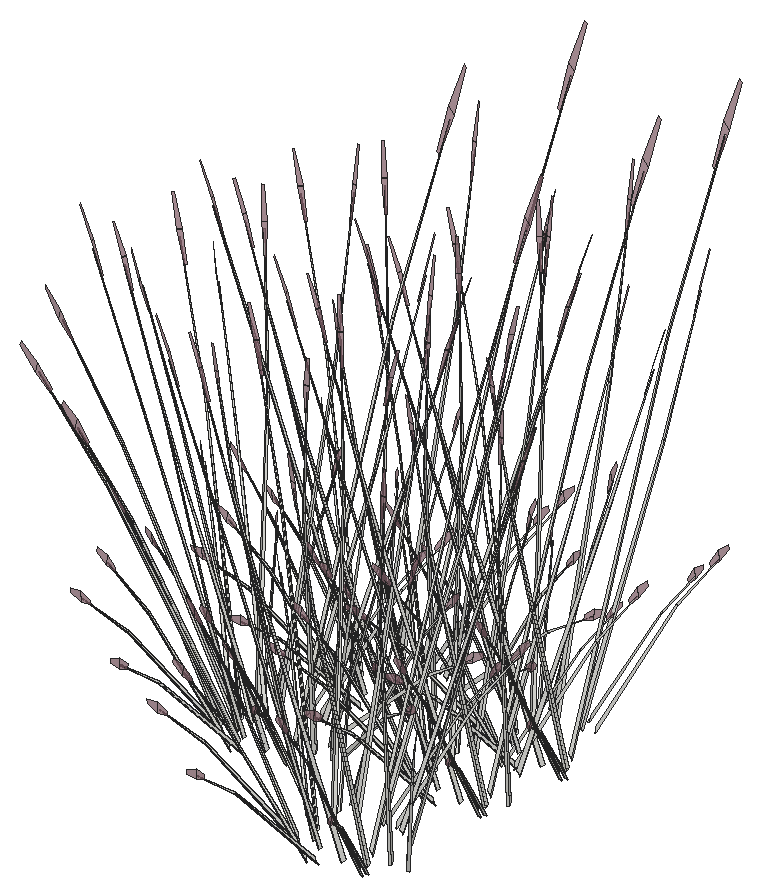
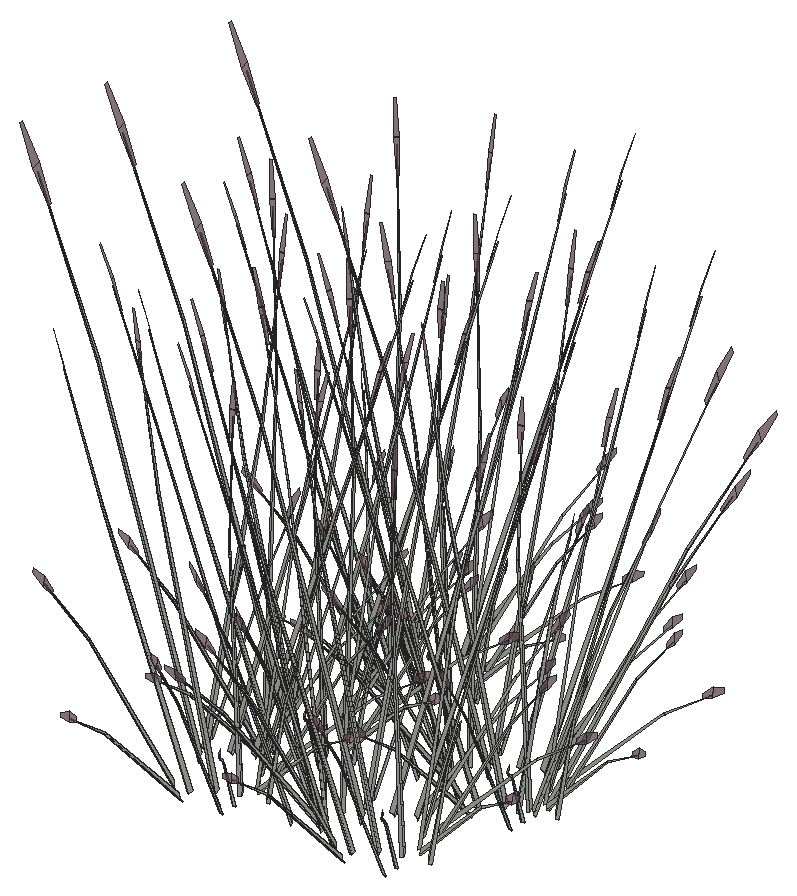
# SketchUp Ruby script. Lengths in inches.
U = 1.inch
M = Sketchup.active_model
def pt(a) = Geom::Point3d.new(a.map { |v| v * U })
def face(e, loops, mat)
  f = e.add_face(loops[0].map { |a| pt(a) })
  loops[1..].each { |l| e.add_face(l.map { |a| pt(a) }).erase! }
  f.material = f.back_material = mat if mat
  f
end
# faces: each face lists its corners as indices into pts; further lists are holes
def faces(e, pts, list, mat = nil) = list.each { |f| face(e, (f[0].is_a?(Array) ? f : [f]).map { |l| l.map { |i| pts[i] } }, mat) }
# xy, xz, yz: faces in a plane at the given z, y or x. An outline is a flat list of corners, or four numbers for a rectangle; further outlines are holes
def ring(l) = l.size == 4 ? [[l[0], l[1]], [l[2], l[1]], [l[2], l[3]], [l[0], l[3]]] : l.each_slice(2).to_a
def flat(e, list, mat, &to3) = list.each { |f| face(e, (f[0].is_a?(Array) ? f : [f]).map { |l| ring(l).map { |u, v| to3.(u, v) } }, mat) }
def xy(e, z, list, mat = nil) = flat(e, list, mat) { |x, y| [x, y, z] }
def xz(e, y, list, mat = nil) = flat(e, list, mat) { |x, z| [x, y, z] }
def yz(e, x, list, mat = nil) = flat(e, list, mat) { |y, z| [x, y, z] }
def lines(e, pts, list) = list.each { |a, b| e.add_line(pt(pts[a]), pt(pts[b])) }
# prism: a flat outline (further loops are holes) pulled along v
def prism(e, loops, v, mat = nil)
  f = face(e, loops, mat); d = Geom::Vector3d.new(v.map { |x| x * U })
  f.pushpull(f.normal.samedirection?(d) ? d.length : -d.length)
end
def box(e, o, s, mat = nil) = prism(e, [[o, [o[0] + s[0], o[1], o[2]], [o[0] + s[0], o[1] + s[1], o[2]], [o[0], o[1] + s[1], o[2]]]], [0, 0, s[2]], mat)
def at(x, y, z, deg = 0) = Geom::Transformation.translation(pt([x, y, z])) * Geom::Transformation.rotation(ORIGIN, Z_AXIS, deg.degrees)
def axes(o, x, y, z) = Geom::Transformation.new([*x, 0, *y, 0, *z, 0, *pt(o).to_a, 1])
def part(name) = M.definitions.add(name)
# library, detail: a bought-in or finely detailed component or shape, given as its bounding box
def library(name, o, s) = part(name).tap { |d| box(d.entities, o, s) }
def detail(e, o, s) = box(e.add_group.entities, o, s)
def put(e, d, t, mat = nil) = e.add_instance(d, t).tap { |i| i.material = mat if mat }
def group(e, t, mat = nil) = e.add_group.tap { |g| g.transformation = t; g.material = mat if mat }.entities
root = M.entities
M.materials.add("LightPink_Translucent").color = [144, 107, 117]
M.materials["LightPink_Translucent"].alpha = 0.75
c1 = part("blade")
p = [[2.15,0.21,22],[0,0.17,0],[0.09,0.45,0],[2.18,0.31,22],[2.29,0.31,22],[0.38,0.45,0],
  [2.48,0.24,33],[2.49,0.24,33],[2.48,0.22,33]]
faces(c1.entities,p,[[0,1,2,3],[4,5,2,3],[6,3,4,7],[8,0,3,6]])
c2 = part("seeds")
p = [[0.3,-0.1,1.38],[-0.01,-0.03,1.59],[-0.01,-0.03,0.03],[0.14,-0.07,-0.07],[0.29,-0.03,3],[0.15,0.01,3.11]]
faces(c2.entities,p,[[0,1,2,3],[1,0,4,5]],"LightPink_Translucent")
c3 = part("blade with seeds")
put(c3.entities,c1,at(0,0,0))
put(c3.entities,c2,axes([2.4,0.25,30.99],[1.5799,-0.05474,1.17369],[-0.12525,1.92788,0.29478],[-0.07173,-0.02425,1.56792]))
put(root,c3,axes([662.58,339.65,513.22],[0.26985,-0.01293,1.42242],[-0.17902,0.56047,0.11501],[-0.38456,-0.03467,0.60807]))
put(root,c3,axes([662.69,340.64,513.22],[0.22574,-0.12077,1.42242],[0.19004,0.55807,0.11501],[-0.35439,0.12613,0.60807]))
put(root,c3,axes([662,340.45,513.91],[-0.10624,0.07413,1.45204],[0.00904,0.54162,-0.22964],[-0.24352,0.07044,0.11645]))
put(root,c3,axes([663.09,338.76,513.22],[0.24166,0.09837,1.42242],[-0.50011,0.41269,0.11501],[-0.3117,-0.18617,0.60807]))
put(root,c3,axes([660.82,340.99,513.91],[0.08303,0.01531,1.47228],[0.25685,0.50448,-0.13912],[-0.16996,0.13241,0.26054]))
put(root,c3,axes([662.5,338.19,513.91],[0.04823,0.05698,1.47228],[-0.23252,0.51221,-0.13912],[-0.23548,0.00371,0.26054]))
put(root,c3,axes([663.04,337.85,513.91],[-0.13998,-0.00403,1.45204],[-0.44565,0.40302,-0.22964],[-0.23779,-0.08235,0.11645]))
put(root,c3,axes([662.68,339.93,514.18],[0.32734,0.51701,-0.10093],[-0.58097,0.25407,-0.56021],[-0.24483,0.06821,0.85122]))
put(root,c3,axes([663.42,338.85,514.18],[-0.03484,0.58066,-0.10093],[-0.65957,-0.01587,-0.56021],[-0.25402,-0.04034,0.85122]))
put(root,c3,axes([663.52,341.02,513.22],[0.1625,-0.17544,1.42242],[0.41029,0.47354,0.11501],[-0.28141,0.21565,0.60807]))
put(root,c3,axes([664.26,348.79,513.91],[-0.10624,0.07413,1.45204],[0.00904,0.54162,-0.22964],[-0.24352,0.07044,0.11645]))
put(root,c3,axes([662.02,342.47,513.91],[-0.01617,0.11299,1.45204],[0.45894,0.39307,-0.22964],[-0.12015,0.18588,0.11645]))
put(root,c3,axes([664.71,338.01,514.51],[-0.4342,0.54737,-0.11304],[-0.6288,-0.31535,-0.62743],[-0.21858,-0.15465,0.95337]))
put(root,c3,axes([663.08,349.33,513.91],[0.08303,0.01531,1.47228],[0.25685,0.50448,-0.13912],[-0.16996,0.13241,0.26054]))
put(root,c3,axes([662.71,341.16,514.18],[0.60181,0.31483,-0.10093],[-0.34671,0.45593,-0.56021],[-0.17003,0.15849,0.85122]))
put(root,c3,axes([664.76,346.53,513.91],[0.04823,0.05698,1.47228],[-0.23252,0.51221,-0.13912],[-0.23548,0.00371,0.26054]))
put(root,c3,axes([665.3,346.19,513.91],[-0.13998,-0.00403,1.45204],[-0.44565,0.40302,-0.22964],[-0.23779,-0.08235,0.11645]))
put(root,c3,axes([664.94,348.27,514.18],[0.32734,0.51701,-0.10093],[-0.58097,0.25407,-0.56021],[-0.24483,0.06821,0.85122]))
put(root,c3,axes([665.68,347.2,514.18],[-0.03484,0.58066,-0.10093],[-0.65957,-0.01587,-0.56021],[-0.25402,-0.04034,0.85122]))
put(root,c3,axes([664.54,336.71,513.91],[-0.01214,0.06844,1.47228],[-0.59861,0.24837,-0.13912],[-0.17615,-0.12696,0.26054]))
put(root,c3,axes([664.09,338.18,513.22],[0.14872,0.18332,1.42242],[-0.6872,0.15433,0.11501],[-0.15531,-0.28779,0.60807]))
put(root,c3,axes([661.97,343.625,513.91],[0.07381,-0.03447,1.47228],[0.61004,0.22929,-0.13912],[-0.01434,0.19091,0.26054]))
put(root,c3,axes([664.28,350.81,513.91],[-0.01617,0.11299,1.45204],[0.45894,0.39307,-0.22964],[-0.12015,0.18588,0.11645]))
put(root,c3,axes([666.96,346.35,514.51],[-0.4342,0.54737,-0.11304],[-0.6288,-0.31535,-0.62743],[-0.21858,-0.15465,0.95337]))
put(root,c3,axes([664.97,349.5,514.18],[0.60181,0.31483,-0.10093],[-0.34671,0.45593,-0.56021],[-0.17003,0.15849,0.85122]))
put(root,c3,axes([665.22,336.97,513.91],[-0.09951,-0.08005,1.45204],[-0.66407,0.05075,-0.22964],[-0.10598,-0.19148,0.11645]))
put(root,c3,axes([666.8,345.05,513.91],[-0.01214,0.06844,1.47228],[-0.59861,0.24837,-0.13912],[-0.17615,-0.12696,0.26054]))
put(root,c3,axes([663.49,342.21,514.48],[0.71502,0.02829,-0.11203],[-0.01954,0.53563,-0.62183],[-0.04967,0.20629,0.94486]))
put(root,c3,axes([666.23,338.2,514.18],[-0.63664,0.26583,-0.10093],[-0.31286,-0.47181,-0.56021],[-0.084,-0.19882,0.85122]))
put(root,c3,axes([664.22,351.97,513.91],[0.07381,-0.03447,1.47228],[0.61004,0.22929,-0.13912],[-0.01434,0.19091,0.26054]))
put(root,c3,axes([667.48,345.31,513.91],[-0.09951,-0.08005,1.45204],[-0.66407,0.05075,-0.22964],[-0.10598,-0.19148,0.11645]))
put(root,c3,axes([665.74,350.55,514.48],[0.71502,0.02829,-0.11203],[-0.01954,0.53563,-0.62183],[-0.04967,0.20629,0.94486]))
put(root,c3,axes([668.49,346.54,514.18],[-0.63664,0.26583,-0.10093],[-0.31286,-0.47181,-0.56021],[-0.084,-0.19882,0.85122]))
put(root,c3,axes([664.66,343.86,513.91],[0.08247,0.09194,1.45204],[0.66552,0.03612,-0.22964],[0.06692,0.20277,0.11645]))
put(root,c3,axes([664.81,342.81,514.18],[0.63664,-0.26583,-0.10093],[0.31286,0.47181,-0.56021],[0.084,0.19882,0.85122]))
put(root,c3,axes([668.0625,337.54,513.91],[-0.06607,0.04361,1.47228],[-0.64734,-0.14714,-0.13912],[-0.02343,-0.19032,0.26054]))
put(root,c3,axes([667.55,338.8,514.18],[-0.71502,-0.02829,-0.10093],[0.01954,-0.53563,-0.56021],[0.04967,-0.20629,0.85122]))
put(root,c3,axes([666.92,352.21,513.91],[0.08247,0.09194,1.45204],[0.66552,0.03612,-0.22964],[0.06692,0.20277,0.11645]))
put(root,c3,axes([673.63,332.98,513.91],[-0.10624,0.07413,1.45204],[0.00904,0.54162,-0.22964],[-0.24352,0.07044,0.11645]))
put(root,c3,axes([666.76,339.91,513.71],[-0.56218,-0.29666,1.14775],[0.59361,-0.46189,0.49522],[0.18138,0.27836,1.10941]))
put(root,c3,axes([665.81,343.2,513.91],[0.00193,-0.06913,1.47228],[0.55753,-0.30498,-0.13912],[0.19366,0.10886,0.26054]))
put(root,c3,axes([672.45,333.53,513.91],[0.08303,0.01531,1.47228],[0.25685,0.50448,-0.13912],[-0.16996,0.13241,0.26054]))
put(root,c3,axes([668.2,337.95,513.91],[-0.00628,-0.11364,1.45204],[-0.53042,-0.32843,-0.22964],[0.08201,-0.19909,0.11645]))
put(root,c3,axes([667.07,351.15,514.18],[0.63664,-0.26583,-0.10093],[0.31286,0.47181,-0.56021],[0.084,0.19882,0.85122]))
put(root,c3,axes([670.32,345.88,513.91],[-0.06607,0.04361,1.47228],[-0.64734,-0.14714,-0.13912],[-0.02343,-0.19032,0.26054]))
put(root,c3,axes([669.8125,347.14,514.18],[-0.71502,-0.02829,-0.10093],[0.01954,-0.53563,-0.56021],[0.04967,-0.20629,0.85122]))
put(root,c3,axes([674.13,330.73,513.91],[0.04823,0.05698,1.47228],[-0.23252,0.51221,-0.13912],[-0.23548,0.00371,0.26054]))
put(root,c3,axes([674.62,342.66,513.91],[-0.10624,0.07413,1.45204],[0.00904,0.54162,-0.22964],[-0.24352,0.07044,0.11645]))
put(root,c3,axes([674.67,330.39,513.91],[-0.13998,-0.00403,1.45204],[-0.44565,0.40302,-0.22964],[-0.23779,-0.08235,0.11645]))
put(root,c3,axes([674.31,332.46,514.18],[0.32734,0.51701,-0.10093],[-0.58097,0.25407,-0.56021],[-0.24483,0.06821,0.85122]))
put(root,c3,axes([675.05,331.39,514.18],[-0.03484,0.58066,-0.10093],[-0.65957,-0.01587,-0.56021],[-0.25402,-0.04034,0.85122]))
put(root,c3,axes([673.44,343.21,513.91],[0.08303,0.01531,1.47228],[0.25685,0.50448,-0.13912],[-0.16996,0.13241,0.26054]))
put(root,c3,axes([666.32,342.79,514.18],[0.38768,-0.48872,-0.10093],[0.56143,0.28156,-0.56021],[0.19516,0.13808,0.85122]))
put(root,c3,axes([668.33,339.85,514.18],[-0.60181,-0.31483,-0.10093],[0.34671,-0.45593,-0.56021],[0.17003,-0.15849,0.85122]))
put(root,c3,axes([675.12,340.4,513.91],[0.04823,0.05698,1.47228],[-0.23252,0.51221,-0.13912],[-0.23548,0.00371,0.26054]))
put(root,c3,axes([675.57,348.99,513.91],[-0.10624,0.07413,1.45204],[0.00904,0.54162,-0.22964],[-0.24352,0.07044,0.11645]))
put(root,c3,axes([675.66,340.0625,513.91],[-0.13998,-0.00403,1.45204],[-0.44565,0.40302,-0.22964],[-0.23779,-0.08235,0.11645]))
put(root,c3,axes([675.3,342.14,514.18],[0.32734,0.51701,-0.10093],[-0.58097,0.25407,-0.56021],[-0.24483,0.06821,0.85122]))
put(root,c3,axes([676.03,341.07,514.18],[-0.03484,0.58066,-0.10093],[-0.65957,-0.01587,-0.56021],[-0.25402,-0.04034,0.85122]))
put(root,c3,axes([674.39,349.54,513.91],[0.08303,0.01531,1.47228],[0.25685,0.50448,-0.13912],[-0.16996,0.13241,0.26054]))
put(root,c3,axes([673.64,335,513.91],[-0.01617,0.11299,1.45204],[0.45894,0.39307,-0.22964],[-0.12015,0.18588,0.11645]))
put(root,c3,axes([669.02,348.25,513.71],[-0.56218,-0.29666,1.14775],[0.59361,-0.46189,0.49522],[0.18138,0.27836,1.10941]))
put(root,c3,axes([676.33,330.54,514.51],[-0.4342,0.54737,-0.11304],[-0.6288,-0.31535,-0.62743],[-0.21858,-0.15465,0.95337]))
put(root,c3,axes([668.07,351.54,513.91],[0.00193,-0.06913,1.47228],[0.55753,-0.30498,-0.13912],[0.19366,0.10886,0.26054]))
put(root,c3,axes([670.46,346.29,513.91],[-0.00628,-0.11364,1.45204],[-0.53042,-0.32843,-0.22964],[0.08201,-0.19909,0.11645]))
put(root,c3,axes([676.07,346.74,513.91],[0.04823,0.05698,1.47228],[-0.23252,0.51221,-0.13912],[-0.23548,0.00371,0.26054]))
put(root,c3,axes([676.61,346.39,513.91],[-0.13998,-0.00403,1.45204],[-0.44565,0.40302,-0.22964],[-0.23779,-0.08235,0.11645]))
put(root,c3,axes([674.33,333.69,514.18],[0.60181,0.31483,-0.10093],[-0.34671,0.45593,-0.56021],[-0.17003,0.15849,0.85122]))
put(root,c3,axes([676.25,348.47,514.18],[0.32734,0.51701,-0.10093],[-0.58097,0.25407,-0.56021],[-0.24483,0.06821,0.85122]))
put(root,c3,axes([669.8125,339.72,513.91],[-0.08498,-0.00434,1.47228],[-0.35287,-0.46464,-0.13912],[0.14171,-0.15278,0.26054]))
put(root,c3,axes([676.98,347.4,514.18],[-0.03484,0.58066,-0.10093],[-0.65957,-0.01587,-0.56021],[-0.25402,-0.04034,0.85122]))
put(root,c3,axes([667.62,342.16,514.18],[0.03484,-0.58066,-0.10093],[0.65957,0.01587,-0.56021],[0.25402,0.04034,0.85122]))
put(root,c3,axes([668.36,341.08,514.18],[-0.32734,-0.51701,-0.10093],[0.58097,-0.25407,-0.56021],[0.24483,-0.06821,0.85122]))
put(root,c3,axes([674.63,344.68,513.91],[-0.01617,0.11299,1.45204],[0.45894,0.39307,-0.22964],[-0.12015,0.18588,0.11645]))
put(root,c3,axes([677.32,340.22,514.51],[-0.4342,0.54737,-0.11304],[-0.6288,-0.31535,-0.62743],[-0.21858,-0.15465,0.95337]))
put(root,c3,axes([668.58,351.13,514.18],[0.38768,-0.48872,-0.10093],[0.56143,0.28156,-0.56021],[0.19516,0.13808,0.85122]))
put(root,c3,axes([676.17,329.24,513.91],[-0.01214,0.06844,1.47228],[-0.59861,0.24837,-0.13912],[-0.17615,-0.12696,0.26054]))
put(root,c3,axes([670.59,348.2,514.18],[-0.60181,-0.31483,-0.10093],[0.34671,-0.45593,-0.56021],[0.17003,-0.15849,0.85122]))
put(root,c3,axes([668.19,341.81,513.91],[0.13956,-0.00966,1.45204],[0.38281,-0.44358,-0.22964],[0.24825,0.05855,0.11645]))
put(root,c3,axes([675.32,343.37,514.18],[0.60181,0.31483,-0.10093],[-0.34671,0.45593,-0.56021],[-0.17003,0.15849,0.85122]))
put(root,c3,axes([675.58,351.01,513.91],[-0.01617,0.11299,1.45204],[0.45894,0.39307,-0.22964],[-0.12015,0.18588,0.11645]))
put(root,c3,axes([678.27,346.55,514.51],[-0.4342,0.54737,-0.11304],[-0.6288,-0.31535,-0.62743],[-0.21858,-0.15465,0.95337]))
put(root,c3,axes([673.59,336.16,513.91],[0.07381,-0.03447,1.47228],[0.61004,0.22929,-0.13912],[-0.01434,0.19091,0.26054]))
put(root,c3,axes([669.66,342.62,513.91],[-0.05883,-0.04999,1.47228],[0.12868,-0.53581,-0.13912],[0.23172,-0.03423,0.26054]))
put(root,c3,axes([677.15,338.92,513.91],[-0.01214,0.06844,1.47228],[-0.59861,0.24837,-0.13912],[-0.17615,-0.12696,0.26054]))
put(root,c3,axes([676.27,349.7,514.18],[0.60181,0.31483,-0.10093],[-0.34671,0.45593,-0.56021],[-0.17003,0.15849,0.85122]))
put(root,c3,axes([670.13,340.27,513.91],[0.09028,-0.08697,1.45204],[-0.11555,-0.53348,-0.22964],[0.22652,-0.10115,0.11645]))
put(root,c3,axes([672.07,348.06,513.91],[-0.08498,-0.00434,1.47228],[-0.35287,-0.46464,-0.13912],[0.14171,-0.15278,0.26054]))
put(root,c3,axes([674.58,345.84,513.91],[0.07381,-0.03447,1.47228],[0.61004,0.22929,-0.13912],[-0.01434,0.19091,0.26054]))
put(root,c3,axes([676.85,329.5,513.91],[-0.09951,-0.08005,1.45204],[-0.66407,0.05075,-0.22964],[-0.10598,-0.19148,0.11645]))
put(root,c3,axes([669.88,350.5,514.18],[0.03484,-0.58066,-0.10093],[0.65957,0.01587,-0.56021],[0.25402,0.04034,0.85122]))
put(root,c3,axes([670.61,349.42,514.18],[-0.32734,-0.51701,-0.10093],[0.58097,-0.25407,-0.56021],[0.24483,-0.06821,0.85122]))
put(root,c3,axes([678.1,345.25,513.91],[-0.01214,0.06844,1.47228],[-0.59861,0.24837,-0.13912],[-0.17615,-0.12696,0.26054]))
put(root,c3,axes([670.45,350.15,513.91],[0.13956,-0.00966,1.45204],[0.38281,-0.44358,-0.22964],[0.24825,0.05855,0.11645]))
put(root,c3,axes([675.11,334.75,514.48],[0.71502,0.02829,-0.11203],[-0.01954,0.53563,-0.62183],[-0.04967,0.20629,0.94486]))
put(root,c3,axes([677.86,330.74,514.18],[-0.63664,0.26583,-0.10093],[-0.31286,-0.47181,-0.56021],[-0.084,-0.19882,0.85122]))
put(root,c3,axes([675.53,352.17,513.91],[0.07381,-0.03447,1.47228],[0.61004,0.22929,-0.13912],[-0.01434,0.19091,0.26054]))
put(root,c3,axes([677.83,339.18,513.91],[-0.09951,-0.08005,1.45204],[-0.66407,0.05075,-0.22964],[-0.10598,-0.19148,0.11645]))
put(root,c3,axes([671.91,350.96,513.91],[-0.05883,-0.04999,1.47228],[0.12868,-0.53581,-0.13912],[0.23172,-0.03423,0.26054]))
put(root,c3,axes([676.1,344.42,514.48],[0.71502,0.02829,-0.11203],[-0.01954,0.53563,-0.62183],[-0.04967,0.20629,0.94486]))
put(root,c3,axes([678.85,340.42,514.18],[-0.63664,0.26583,-0.10093],[-0.31286,-0.47181,-0.56021],[-0.084,-0.19882,0.85122]))
put(root,c3,axes([678.79,345.51,513.91],[-0.09951,-0.08005,1.45204],[-0.66407,0.05075,-0.22964],[-0.10598,-0.19148,0.11645]))
put(root,c3,axes([672.39,348.61,513.91],[0.09028,-0.08697,1.45204],[-0.11555,-0.53348,-0.22964],[0.22652,-0.10115,0.11645]))
put(root,c3,axes([677.05,350.76,514.48],[0.71502,0.02829,-0.11203],[-0.01954,0.53563,-0.62183],[-0.04967,0.20629,0.94486]))
put(root,c3,axes([679.8,346.75,514.18],[-0.63664,0.26583,-0.10093],[-0.31286,-0.47181,-0.56021],[-0.084,-0.19882,0.85122]))
put(root,c3,axes([676.29,336.4,513.91],[0.08247,0.09194,1.45204],[0.66552,0.03612,-0.22964],[0.06692,0.20277,0.11645]))
put(root,c3,axes([677.27,346.08,513.91],[0.08247,0.09194,1.45204],[0.66552,0.03612,-0.22964],[0.06692,0.20277,0.11645]))
put(root,c3,axes([676.44,335.35,514.18],[0.63664,-0.26583,-0.10093],[0.31286,0.47181,-0.56021],[0.084,0.19882,0.85122]))
put(root,c3,axes([679.6875,330.08,513.91],[-0.06607,0.04361,1.47228],[-0.64734,-0.14714,-0.13912],[-0.02343,-0.19032,0.26054]))
put(root,c3,axes([679.18,331.34,514.18],[-0.71502,-0.02829,-0.10093],[0.01954,-0.53563,-0.56021],[0.04967,-0.20629,0.85122]))
put(root,c3,axes([678.22,352.41,513.91],[0.08247,0.09194,1.45204],[0.66552,0.03612,-0.22964],[0.06692,0.20277,0.11645]))
put(root,c3,axes([677.42,345.02,514.18],[0.63664,-0.26583,-0.10093],[0.31286,0.47181,-0.56021],[0.084,0.19882,0.85122]))
put(root,c3,axes([680.68,339.75,513.91],[-0.06607,0.04361,1.47228],[-0.64734,-0.14714,-0.13912],[-0.02343,-0.19032,0.26054]))
put(root,c3,axes([680.17,341.01,514.18],[-0.71502,-0.02829,-0.10093],[0.01954,-0.53563,-0.56021],[0.04967,-0.20629,0.85122]))
put(root,c3,axes([678.375,351.35,514.18],[0.63664,-0.26583,-0.10093],[0.31286,0.47181,-0.56021],[0.084,0.19882,0.85122]))
put(root,c3,axes([681.63,346.09,513.91],[-0.06607,0.04361,1.47228],[-0.64734,-0.14714,-0.13912],[-0.02343,-0.19032,0.26054]))
put(root,c3,axes([678.39,332.44,513.71],[-0.56218,-0.29666,1.14775],[0.59361,-0.46189,0.49522],[0.18138,0.27836,1.10941]))
put(root,c3,axes([681.12,347.34,514.18],[-0.71502,-0.02829,-0.10093],[0.01954,-0.53563,-0.56021],[0.04967,-0.20629,0.85122]))
put(root,c3,axes([677.44,335.73,513.91],[0.00193,-0.06913,1.47228],[0.55753,-0.30498,-0.13912],[0.19366,0.10886,0.26054]))
put(root,c3,axes([679.83,330.49,513.91],[-0.00628,-0.11364,1.45204],[-0.53042,-0.32843,-0.22964],[0.08201,-0.19909,0.11645]))
put(root,c3,axes([679.375,342.12,513.71],[-0.56218,-0.29666,1.14775],[0.59361,-0.46189,0.49522],[0.18138,0.27836,1.10941]))
put(root,c3,axes([678.43,345.41,513.91],[0.00193,-0.06913,1.47228],[0.55753,-0.30498,-0.13912],[0.19366,0.10886,0.26054]))
put(root,c3,axes([677.95,335.33,514.18],[0.38768,-0.48872,-0.10093],[0.56143,0.28156,-0.56021],[0.19516,0.13808,0.85122]))
put(root,c3,axes([680.82,340.16,513.91],[-0.00628,-0.11364,1.45204],[-0.53042,-0.32843,-0.22964],[0.08201,-0.19909,0.11645]))
put(root,c3,axes([679.96,332.39,514.18],[-0.60181,-0.31483,-0.10093],[0.34671,-0.45593,-0.56021],[0.17003,-0.15849,0.85122]))
put(root,c3,axes([680.33,348.45,513.71],[-0.56218,-0.29666,1.14775],[0.59361,-0.46189,0.49522],[0.18138,0.27836,1.10941]))
put(root,c3,axes([679.38,351.74,513.91],[0.00193,-0.06913,1.47228],[0.55753,-0.30498,-0.13912],[0.19366,0.10886,0.26054]))
put(root,c3,axes([681.77,346.49,513.91],[-0.00628,-0.11364,1.45204],[-0.53042,-0.32843,-0.22964],[0.08201,-0.19909,0.11645]))
put(root,c3,axes([678.9375,345,514.18],[0.38768,-0.48872,-0.10093],[0.56143,0.28156,-0.56021],[0.19516,0.13808,0.85122]))
put(root,c3,axes([680.95,342.07,514.18],[-0.60181,-0.31483,-0.10093],[0.34671,-0.45593,-0.56021],[0.17003,-0.15849,0.85122]))
put(root,c3,axes([681.4375,332.25,513.91],[-0.08498,-0.00434,1.47228],[-0.35287,-0.46464,-0.13912],[0.14171,-0.15278,0.26054]))
put(root,c3,axes([679.25,334.69,514.18],[0.03484,-0.58066,-0.10093],[0.65957,0.01587,-0.56021],[0.25402,0.04034,0.85122]))
